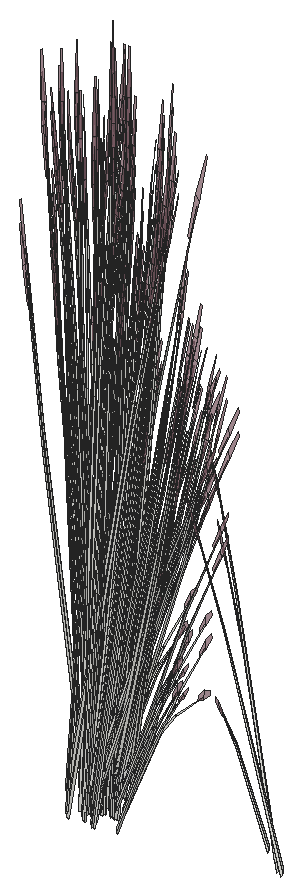
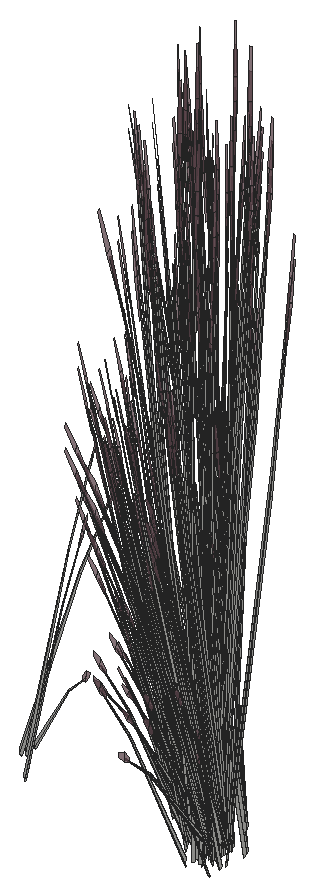
# SketchUp Ruby script. Lengths in inches.
U = 1.inch
M = Sketchup.active_model
def pt(a) = Geom::Point3d.new(a.map { |v| v * U })
def face(e, loops, mat)
  f = e.add_face(loops[0].map { |a| pt(a) })
  loops[1..].each { |l| e.add_face(l.map { |a| pt(a) }).erase! }
  f.material = f.back_material = mat if mat
  f
end
# faces: each face lists its corners as indices into pts; further lists are holes
def faces(e, pts, list, mat = nil) = list.each { |f| face(e, (f[0].is_a?(Array) ? f : [f]).map { |l| l.map { |i| pts[i] } }, mat) }
# xy, xz, yz: faces in a plane at the given z, y or x. An outline is a flat list of corners, or four numbers for a rectangle; further outlines are holes
def ring(l) = l.size == 4 ? [[l[0], l[1]], [l[2], l[1]], [l[2], l[3]], [l[0], l[3]]] : l.each_slice(2).to_a
def flat(e, list, mat, &to3) = list.each { |f| face(e, (f[0].is_a?(Array) ? f : [f]).map { |l| ring(l).map { |u, v| to3.(u, v) } }, mat) }
def xy(e, z, list, mat = nil) = flat(e, list, mat) { |x, y| [x, y, z] }
def xz(e, y, list, mat = nil) = flat(e, list, mat) { |x, z| [x, y, z] }
def yz(e, x, list, mat = nil) = flat(e, list, mat) { |y, z| [x, y, z] }
def lines(e, pts, list) = list.each { |a, b| e.add_line(pt(pts[a]), pt(pts[b])) }
# prism: a flat outline (further loops are holes) pulled along v
def prism(e, loops, v, mat = nil)
  f = face(e, loops, mat); d = Geom::Vector3d.new(v.map { |x| x * U })
  f.pushpull(f.normal.samedirection?(d) ? d.length : -d.length)
end
def box(e, o, s, mat = nil) = prism(e, [[o, [o[0] + s[0], o[1], o[2]], [o[0] + s[0], o[1] + s[1], o[2]], [o[0], o[1] + s[1], o[2]]]], [0, 0, s[2]], mat)
def at(x, y, z, deg = 0) = Geom::Transformation.translation(pt([x, y, z])) * Geom::Transformation.rotation(ORIGIN, Z_AXIS, deg.degrees)
def axes(o, x, y, z) = Geom::Transformation.new([*x, 0, *y, 0, *z, 0, *pt(o).to_a, 1])
def part(name) = M.definitions.add(name)
# library, detail: a bought-in or finely detailed component or shape, given as its bounding box
def library(name, o, s) = part(name).tap { |d| box(d.entities, o, s) }
def detail(e, o, s) = box(e.add_group.entities, o, s)
def put(e, d, t, mat = nil) = e.add_instance(d, t).tap { |i| i.material = mat if mat }
def group(e, t, mat = nil) = e.add_group.tap { |g| g.transformation = t; g.material = mat if mat }.entities
root = M.entities
M.materials.add("LightPink_Translucent").color = [144, 107, 117]
M.materials["LightPink_Translucent"].alpha = 0.75
c1 = part("blade")
p = [[2.15,0.21,22],[0,0.17,0],[0.09,0.45,0],[2.18,0.31,22],[2.29,0.31,22],[0.38,0.45,0],
  [2.48,0.24,33],[2.49,0.24,33],[2.48,0.22,33]]
faces(c1.entities,p,[[0,1,2,3],[4,5,2,3],[6,3,4,7],[8,0,3,6]])
c2 = part("seeds")
p = [[0.3,-0.1,1.38],[-0.01,-0.03,1.59],[-0.01,-0.03,0.03],[0.14,-0.07,-0.07],[0.29,-0.03,3],[0.15,0.01,3.11]]
faces(c2.entities,p,[[0,1,2,3],[1,0,4,5]],"LightPink_Translucent")
c3 = part("blade with seeds")
put(c3.entities,c1,at(0,0,0))
put(c3.entities,c2,axes([2.4,0.25,30.99],[1.5799,-0.05474,1.17369],[-0.12525,1.92788,0.29478],[-0.07173,-0.02425,1.56792]))
put(root,c3,axes([274.08,462.69,652.73],[-0.35779,-0.36745,0.48003],[0.37996,-0.3169,0.3958],[-0.066,0.17239,0.9933]))
put(root,c3,axes([274.34,462.3125,650.03],[-0.11803,-0.46926,-0.30978],[0.46876,-0.13325,0.30978],[-0.0945,-0.05411,1.38974]))
put(root,c3,axes([274.34,462.3125,652.03],[-0.11803,-0.46926,-0.30978],[0.46876,-0.13325,0.30978],[-0.0945,-0.05411,1.38974]))
put(root,c3,axes([273.95,462.66,652.73],[-0.4129,-0.02509,0.0643],[0.01132,-0.37891,0.50621],[-0.04321,0.14514,0.77189]))
put(root,c3,axes([274.08,462.8,652.53],[-0.33997,0.28354,-0.35414],[-0.32182,-0.32376,0.4572],[-0.04897,0.1645,0.87481]))
put(root,c3,axes([274.08,462.8,654.53],[-0.33997,0.28354,-0.35414],[-0.32182,-0.32376,0.4572],[-0.04897,0.1645,0.87481]))
put(root,c3,axes([275.82,461.95,650.06],[-0.33843,0.40479,-0.62353],[-0.42041,-0.36705,-0.16365],[-0.13561,0.10098,1.37633]))
put(root,c3,axes([275.82,461.95,652.06],[-0.33843,0.40479,-0.62353],[-0.42041,-0.36705,-0.16365],[-0.13561,0.10098,1.37633]))
put(root,c3,axes([272.87,463.8125,652.71],[0.057,-0.03251,1.77383],[0.47114,0.21627,-0.16761],[-0.01107,0.18007,0.31391]))
put(root,c3,axes([276.05,461.73,650.46],[-0.49063,-0.43346,-0.25192],[0.41285,-0.48673,0.5513],[-0.13212,0.05071,1.68216]))
put(root,c3,axes([276.05,461.73,652.46],[-0.49063,-0.43346,-0.25192],[0.41285,-0.48673,0.5513],[-0.13212,0.05071,1.68216]))
put(root,c3,axes([274.31,462.5,653.34],[-0.01307,0.49815,-0.7886],[-0.55054,-0.03346,0.09517],[-0.0581,0.21104,1.11556]))
put(root,c3,axes([274.31,462.5,655.34],[-0.01307,0.49815,-0.7886],[-0.55054,-0.03346,0.09517],[-0.0581,0.21104,1.11556]))
put(root,c3,axes([274.3,463.9,650.77],[-0.013,-0.32022,1.1486],[0.32493,0.22839,0.84392],[-0.0639,0.15263,0.25299]))
put(root,c3,axes([274.3,463.9,652.77],[-0.013,-0.32022,1.1486],[0.32493,0.22839,0.84392],[-0.0639,0.15263,0.25299]))
put(root,c3,axes([275.8,461.63,650.21],[-0.54562,0.03324,-0.44739],[-0.04934,-0.55185,0.21531],[-0.09768,0.05593,1.43643]))
put(root,c3,axes([275.8,461.63,652.21],[-0.54562,0.03324,-0.44739],[-0.04934,-0.55185,0.21531],[-0.09768,0.05593,1.43643]))
put(root,c3,axes([274.76,462.56,650.48],[0.47024,0.26927,0.49651],[-0.28107,0.48284,0],[-0.1071,-0.06133,1.57504]))
put(root,c3,axes([274.76,462.56,652.48],[0.47024,0.26927,0.49651],[-0.28107,0.48284,0],[-0.1071,-0.06133,1.57504]))
put(root,c3,axes([274.12,463.2,651.36],[0.01104,-0.27801,1.54345],[0.49652,0.14685,0.21329],[-0.04302,0.2963,0.72882]))
put(root,c3,axes([274.12,463.2,653.36],[0.01104,-0.27801,1.54345],[0.49652,0.14685,0.21329],[-0.04302,0.2963,0.72882]))
put(root,c3,axes([275.44,461.72,650.62],[-0.09693,0.48062,0.1448],[-0.47357,-0.08343,-0.41347],[-0.08619,-0.04935,1.26744]))
put(root,c3,axes([275.44,461.72,652.62],[-0.09693,0.48062,0.1448],[-0.47357,-0.08343,-0.41347],[-0.08619,-0.04935,1.26744]))
put(root,c3,axes([276.38,463.06,650.02],[-0.47024,0.26927,-0.49651],[-0.28107,-0.48284,0],[-0.1071,0.06133,1.57504]))
put(root,c3,axes([276.38,463.06,652.02],[-0.47024,0.26927,-0.49651],[-0.28107,-0.48284,0],[-0.1071,0.06133,1.57504]))
put(root,c3,axes([276.41,462.91,650.19],[-0.31023,-0.54153,-0.05142],[0.52557,-0.30095,0.51607],[-0.12951,0.05156,1.6363]))
put(root,c3,axes([276.41,462.91,652.19],[-0.31023,-0.54153,-0.05142],[0.52557,-0.30095,0.51607],[-0.12951,0.05156,1.6363]))
put(root,c3,axes([274.42,462.67,653],[0.35968,0.36185,-0.5672],[-0.37996,0.3169,-0.43934],[-0.05473,0.18385,1.08528]))
put(root,c3,axes([274.42,462.67,655],[0.35968,0.36185,-0.5672],[-0.37996,0.3169,-0.43934],[-0.05473,0.18385,1.08528]))
put(root,c3,axes([276.27,462.84,650.03],[-0.46876,-0.13325,-0.30978],[0.11803,-0.46926,0.30978],[-0.0945,0.05411,1.38974]))
put(root,c3,axes([276.27,462.84,652.03],[-0.46876,-0.13325,-0.30978],[0.11803,-0.46926,0.30978],[-0.0945,0.05411,1.38974]))
put(root,c3,axes([274.26,462.4,653.05],[0.33997,-0.28354,0.35414],[0.32182,0.32376,-0.4572],[-0.04897,0.1645,0.87481]))
put(root,c3,axes([276.54,460.84,650.84],[-0.01373,-0.50706,1.41272],[0.62119,0.13144,0.59816],[-0.14692,0.27746,1.3335]))
put(root,c3,axes([276.54,460.84,652.84],[-0.01373,-0.50706,1.41272],[0.62119,0.13144,0.59816],[-0.14692,0.27746,1.3335]))
put(root,c3,axes([274.04,462.48,653.4],[0.55221,0.02668,-0.13498],[-0.01509,0.50521,-0.74919],[-0.03836,0.19458,1.13838]))
put(root,c3,axes([274.03,463.21,650.82],[0.45645,-0.09537,0.06507],[0.10494,0.38421,-0.86304],[-0.02894,0.19449,0.7736]))
put(root,c3,axes([274.03,463.21,652.82],[0.45645,-0.09537,0.06507],[0.10494,0.38421,-0.86304],[-0.02894,0.19449,0.7736]))
put(root,c3,axes([276.1875,461.48,650.67],[0.05855,0.61451,-0.29095],[-0.60981,0.03716,-0.50002],[-0.10738,0.08185,1.59708]))
put(root,c3,axes([276.1875,461.48,652.67],[0.05855,0.61451,-0.29095],[-0.60981,0.03716,-0.50002],[-0.10738,0.08185,1.59708]))
put(root,c3,axes([274.83,462.15,651.875],[-0.0123,-0.2067,1.71376],[0.53301,0.13712,0.13857],[-0.03297,0.29456,0.73262]))
put(root,c3,axes([274.83,462.15,653.875],[-0.0123,-0.2067,1.71376],[0.53301,0.13712,0.13857],[-0.03297,0.29456,0.73262]))
put(root,c3,axes([275.28,461.26,650.36],[0.63506,0.11347,0.45755],[-0.12924,0.64083,0.17955],[-0.09281,-0.06188,1.58856]))
put(root,c3,axes([275.28,461.26,652.36],[0.63506,0.11347,0.45755],[-0.12924,0.64083,0.17955],[-0.09281,-0.06188,1.58856]))
put(root,c3,axes([275.11,461.14,650.72],[-0.24378,0.48527,0.44739],[-0.50654,-0.23354,-0.21531],[0,-0.11186,1.43643]))
put(root,c3,axes([275.11,461.14,652.72],[-0.24378,0.48527,0.44739],[-0.50654,-0.23354,-0.21531],[0,-0.11186,1.43643]))
put(root,c3,axes([274.9375,462.28,650.47],[0.53992,-0.14294,0.17642],[0.13332,0.53195,0.35086],[-0.04815,-0.07751,1.60407]))
put(root,c3,axes([274.9375,462.28,652.47],[0.53992,-0.14294,0.17642],[0.13332,0.53195,0.35086],[-0.04815,-0.07751,1.60407]))
put(root,c3,axes([275.63,462.37,650.2],[-0.50654,-0.24178,0],[0.24378,-0.50239,0],[0,0,1.62707]))
put(root,c3,axes([275.63,462.37,652.2],[-0.50654,-0.24178,0],[0.24378,-0.50239,0],[0,0,1.62707]))
put(root,c3,axes([276.8,462.97,650.375],[0.31414,0.53965,0],[-0.52557,0.30095,-0.51607],[-0.1197,0.06854,1.63711]))
put(root,c3,axes([276.8,462.97,652.375],[0.31414,0.53965,0],[-0.52557,0.30095,-0.51607],[-0.1197,0.06854,1.63711]))
put(root,c3,axes([275.21,463.21,653.0625],[-0.4951,-0.14079,0.53283],[0.1693,-0.46287,0.43934],[0.02975,0.18203,1.10256]))
put(root,c3,axes([275.07,463.24,652.73],[-0.37023,0.18303,0.0643],[-0.18122,-0.33376,0.50621],[0.03575,0.14712,0.77189]))
put(root,c3,axes([276.54,462.3125,650.47],[0.14515,-0.53522,0.17642],[0.53115,0.15146,0.35086],[-0.09175,0.00261,1.60407]))
put(root,c3,axes([276.54,462.3125,652.47],[0.14515,-0.53522,0.17642],[0.53115,0.15146,0.35086],[-0.09175,0.00261,1.60407]))
put(root,c3,axes([276.3,461.6,650.62],[0.37121,0.32357,0.1448],[-0.30963,0.36505,-0.41347],[-0.08619,0.04935,1.26744]))
put(root,c3,axes([276.3,461.6,652.62],[0.37121,0.32357,0.1448],[-0.30963,0.36505,-0.41347],[-0.08619,0.04935,1.26744]))
put(root,c3,axes([276.17,461.2,650.3],[-0.46736,-0.46353,-0.06131],[0.46764,-0.46381,0],[-0.01632,-0.01619,1.75571]))
put(root,c3,axes([276.17,461.2,652.3],[-0.46736,-0.46353,-0.06131],[0.46764,-0.46381,0],[-0.01632,-0.01619,1.75571]))
put(root,c3,axes([276.29,461.37,650.72],[0.54562,-0.03324,0.44739],[0.04934,0.55185,-0.21531],[-0.09768,0.05593,1.43643]))
put(root,c3,axes([276.29,461.37,652.72],[0.54562,-0.03324,0.44739],[0.04934,0.55185,-0.21531],[-0.09768,0.05593,1.43643]))
put(root,c3,axes([276.42,462.63,650.33],[0.62903,0.17504,0.30756],[-0.15737,0.62568,-0.36492],[-0.10411,0.07831,1.64885]))
put(root,c3,axes([276.42,462.63,652.33],[0.62903,0.17504,0.30756],[-0.15737,0.62568,-0.36492],[-0.10411,0.07831,1.64885]))
put(root,c3,axes([276.69,462.6,650.48],[0.47024,-0.26927,0.49651],[0.28107,0.48284,0],[-0.1071,0.06133,1.57504]))
put(root,c3,axes([276.69,462.6,652.48],[0.47024,-0.26927,0.49651],[0.28107,0.48284,0],[-0.1071,0.06133,1.57504]))
put(root,c3,axes([275.75,462.16,650.2],[-0.16394,-0.4643,0],[0.46814,-0.1626,0],[0,0,1.54371]))
put(root,c3,axes([275.75,462.16,652.2],[-0.16394,-0.4643,0],[0.46814,-0.1626,0],[0,0,1.54371]))
put(root,c3,axes([275.15,463.14,649.49],[0.08132,-0.0293,1.76342],[0.48914,0.1613,-0.26939],[0.0143,0.18179,0.30037]))
put(root,c3,axes([275.15,463.14,651.49],[0.08132,-0.0293,1.76342],[0.48914,0.1613,-0.26939],[0.0143,0.18179,0.30037]))
put(root,c3,axes([275.26,463.3,652.53],[-0.15148,0.41415,-0.35414],[-0.44193,-0.12079,0.4572],[0.04052,0.16674,0.87481]))
put(root,c3,axes([275.26,463.3,654.53],[-0.15148,0.41415,-0.35414],[-0.44193,-0.12079,0.4572],[0.04052,0.16674,0.87481]))
put(root,c3,axes([276.41,461.24,650.21],[-0.24378,0.48527,-0.44739],[-0.50654,-0.23354,0.21531],[0,0.11186,1.43643]))
put(root,c3,axes([276.41,461.24,652.21],[-0.24378,0.48527,-0.44739],[-0.50654,-0.23354,0.21531],[0,0.11186,1.43643]))
put(root,c3,axes([274.95,464.04,652.72],[0.06369,0.08672,1.74944],[0.51399,0.03407,-0.27667],[0.05169,0.19126,0.14031]))
put(root,c3,axes([277.375,460.95,650.47],[-0.39477,-0.39228,0.17642],[0.39783,-0.38049,0.35086],[-0.0436,0.08011,1.60407]))
put(root,c3,axes([277.375,460.95,652.47],[-0.39477,-0.39228,0.17642],[0.39783,-0.38049,0.35086],[-0.0436,0.08011,1.60407]))
put(root,c3,axes([276.01,460.72,650.21],[0,-0.62313,0],[0.62828,0,0],[0,0,1.79456]))
put(root,c3,axes([276.01,460.72,652.21],[0,-0.62313,0],[0.62828,0,0],[0,0,1.79456]))
put(root,c3,axes([276.33,460.97,650.29],[0,0.62282,-0.05637],[-0.62828,0,0],[0,0.01957,1.79368]))
put(root,c3,axes([276.33,460.97,652.29],[0,0.62282,-0.05637],[-0.62828,0,0],[0,0.01957,1.79368]))
put(root,c3,axes([275.21,462.87,653.05],[0.15148,-0.41415,0.35414],[0.44193,0.12079,-0.4572],[0.04052,0.16674,0.87481]))
put(root,c3,axes([274.99,459.52,650.47],[-0.14515,0.53522,0.17642],[-0.53115,-0.15146,0.35086],[0.09175,-0.00261,1.60407]))
put(root,c3,axes([274.99,459.52,652.47],[-0.14515,0.53522,0.17642],[-0.53115,-0.15146,0.35086],[0.09175,-0.00261,1.60407]))
put(root,c3,axes([276.03,462.18,650.29],[0.21845,0.61869,-0.06012],[-0.62418,0.21679,0],[0.00763,0.02161,1.72173]))
put(root,c3,axes([276.03,462.18,652.29],[0.21845,0.61869,-0.06012],[-0.62418,0.21679,0],[0.00763,0.02161,1.72173]))
put(root,c3,axes([275.31,462.93,652.98],[0.23981,0.43789,-0.71045],[-0.49365,0.24404,0.08574],[0.05608,0.21158,1.00501]))
put(root,c3,axes([275.31,462.93,654.98],[0.23981,0.43789,-0.71045],[-0.49365,0.24404,0.08574],[0.05608,0.21158,1.00501]))
put(root,c3,axes([277.83,461.36,650.2],[-0.62797,-0.00431,-0.04976],[0,-0.6019,0.49943],[-0.01973,0.13702,1.58352]))
put(root,c3,axes([277.83,461.36,652.2],[-0.62797,-0.00431,-0.04976],[0,-0.6019,0.49943],[-0.01973,0.13702,1.58352]))
put(root,c3,axes([276.6,459.55,650.47],[-0.53992,0.14294,0.17642],[-0.13332,-0.53195,0.35086],[0.04815,0.07751,1.60407]))
put(root,c3,axes([276.6,459.55,652.47],[-0.53992,0.14294,0.17642],[-0.13332,-0.53195,0.35086],[0.04815,0.07751,1.60407]))
put(root,c3,axes([275.81,464.34,653.65],[0.34721,-0.30895,-0.06488],[0.31814,0.33837,-0.29416],[0.0224,0.09588,0.97024]))
put(root,c3,axes([275.71,460.33,650.36],[-0.4166,0.48873,0.45755],[-0.49494,-0.43142,0.17955],[0.10044,-0.04877,1.58856]))
put(root,c3,axes([275.71,460.33,652.36],[-0.4166,0.48873,0.45755],[-0.49494,-0.43142,0.17955],[0.10044,-0.04877,1.58856]))
put(root,c3,axes([276.42,461.1,650.21],[0.35073,0.34786,0],[-0.35073,0.34786,0],[0,0,1.69266]))
put(root,c3,axes([276.42,461.1,652.21],[0.35073,0.34786,0],[-0.35073,0.34786,0],[0,0,1.69266]))
put(root,c3,axes([276.42,460.69,650.72],[0.24378,-0.48527,0.44739],[0.50654,0.23354,-0.21531],[0,0.11186,1.43643]))
put(root,c3,axes([276.42,460.69,652.72],[0.24378,-0.48527,0.44739],[0.50654,0.23354,-0.21531],[0,0.11186,1.43643]))
put(root,c3,axes([276.21,462.38,650.2],[0.50654,0.24178,0],[-0.24378,0.50239,0],[0,0,1.74954]))
put(root,c3,axes([276.21,462.38,652.2],[0.50654,0.24178,0],[-0.24378,0.50239,0],[0,0,1.74954]))
put(root,c3,axes([275.49,463.02,652.68],[0.49392,0.135,-0.51099],[-0.1693,0.46287,-0.3958],[0.04529,0.18636,0.97773]))
put(root,c3,axes([275.49,463.02,654.68],[0.49392,0.135,-0.51099],[-0.1693,0.46287,-0.3958],[0.04529,0.18636,0.97773]))
put(root,c3,axes([275.0625,463.04,653.03],[0.49168,-0.25073,-0.1216],[0.24162,0.44501,-0.67495],[0.06487,0.18753,1.02557]))
put(root,c3,axes([276.25,460.58,650.38],[-0.63506,-0.11347,0.49198],[0.12924,-0.64083,0.19306],[0.09281,0.06188,1.70813]))
put(root,c3,axes([276.25,460.58,652.38],[-0.63506,-0.11347,0.49198],[0.12924,-0.64083,0.19306],[0.09281,0.06188,1.70813]))
put(root,c3,axes([277.7,461.45,650.03],[-0.35073,0.33601,-0.30978],[-0.35073,-0.33601,0.30978],[0,0.10823,1.38974]))
put(root,c3,axes([277.7,461.45,652.03],[-0.35073,0.33601,-0.30978],[-0.35073,-0.33601,0.30978],[0,0.10823,1.38974]))
put(root,c3,axes([276.7,461.39,650.09],[0.18424,0.49308,-0.69212],[-0.53071,0.17758,-0.18165],[0.02036,0.16697,1.52773]))
put(root,c3,axes([276.7,461.39,652.09],[0.18424,0.49308,-0.69212],[-0.53071,0.17758,-0.18165],[0.02036,0.16697,1.52773]))
put(root,c3,axes([276.4375,460.86,650.21],[0.56215,0,0],[0,0.55754,0],[0,0,1.78407]))
put(root,c3,axes([276.4375,460.86,652.21],[0.56215,0,0],[0,0.55754,0],[0,0,1.78407]))
put(root,c3,axes([275.9,460.25,650.72],[-0.30184,-0.45202,0.44739],[0.45719,-0.31831,-0.21531],[0.09768,0.05593,1.43643]))
put(root,c3,axes([275.9,460.25,652.72],[-0.30184,-0.45202,0.44739],[0.45719,-0.31831,-0.21531],[0.09768,0.05593,1.43643]))
put(root,c3,axes([276.63,460.8,650.62],[0.46814,-0.15705,0.1448],[0.16394,0.44848,-0.41347],[0,0.0987,1.26744]))
put(root,c3,axes([276.63,460.8,652.62],[0.46814,-0.15705,0.1448],[0.16394,0.44848,-0.41347],[0,0.0987,1.26744]))
put(root,c3,axes([276.47,460.84,650.67],[0.56585,0.25696,-0.29095],[-0.27246,0.54236,-0.50002],[0.01778,0.13316,1.59708]))
put(root,c3,axes([276.47,460.84,652.67],[0.56585,0.25696,-0.29095],[-0.27246,0.54236,-0.50002],[0.01778,0.13316,1.59708]))
put(root,c3,axes([277.7,460.96,650.48],[0,-0.53854,0.49651],[0.56215,0,0],[0,0.12266,1.57504]))
put(root,c3,axes([277.7,460.96,652.48],[0,-0.53854,0.49651],[0.56215,0,0],[0,0.12266,1.57504]))
put(root,c3,axes([277.94,461.46,650.02],[0,0.53854,-0.49651],[-0.56215,0,0],[0,0.12266,1.57504]))
put(root,c3,axes([277.94,461.46,652.02],[0,0.53854,-0.49651],[-0.56215,0,0],[0,0.12266,1.57504]))
put(root,c3,axes([276.4375,463.09,652.73],[-0.49974,0.12359,0.48003],[-0.08673,-0.48481,0.3958],[0.11753,0.14288,0.9933]))
put(root,c3,axes([276.34,463.19,652.73],[-0.22836,0.34211,0.0643],[-0.3252,-0.19918,0.50621],[0.10513,0.10968,0.77189]))
put(root,c3,axes([275.77,462.0625,651.875],[-0.11485,-0.17291,1.71376],[0.53072,-0.14557,0.13857],[0.11995,0.27145,0.73262]))
put(root,c3,axes([275.77,462.0625,653.875],[-0.11485,-0.17291,1.71376],[0.53072,-0.14557,0.13857],[0.11995,0.27145,0.73262]))
put(root,c3,axes([276.1,460.12,650.62],[0.09693,-0.48062,0.1448],[0.47357,0.08343,-0.41347],[0.08619,0.04935,1.26744]))
put(root,c3,axes([276.1,460.12,652.62],[0.09693,-0.48062,0.1448],[0.47357,0.08343,-0.41347],[0.08619,0.04935,1.26744]))
put(root,c3,axes([276.77,459.28,650.48],[-0.47024,-0.26927,0.49651],[0.28107,-0.48284,0],[0.1071,0.06133,1.57504]))
put(root,c3,axes([276.77,459.28,652.48],[-0.47024,-0.26927,0.49651],[0.28107,-0.48284,0],[0.1071,0.06133,1.57504]))
put(root,c3,axes([276.36,462.09,650.18],[0.5275,-0.18273,-0.19198],[0.18536,0.52636,0.00008],[0.05823,-0.0202,1.73897]))
put(root,c3,axes([276.36,462.09,652.18],[0.5275,-0.18273,-0.19198],[0.18536,0.52636,0.00008],[0.05823,-0.0202,1.73897]))
put(root,c3,axes([276.27,462.8,653.05],[-0.0776,-0.43378,0.35414],[0.44361,-0.11454,-0.4572],[0.11915,0.12431,0.87481]))
put(root,c3,axes([276.37,460.53,650.21],[0.30184,0.45202,-0.44739],[-0.45719,0.31831,0.21531],[0.09768,0.05593,1.43643]))
put(root,c3,axes([276.37,460.53,652.21],[0.30184,0.45202,-0.44739],[-0.45719,0.31831,0.21531],[0.09768,0.05593,1.43643]))
put(root,c3,axes([276.57,460.3,652.47],[-0.43417,-0.27982,1.38283],[0.45844,-0.43566,0.59665],[0.14008,0.26255,1.33663]))
put(root,c3,axes([275.84,463.4,652.71],[0.00149,-0.0652,1.77383],[0.43058,-0.28766,-0.16761],[0.14956,0.10267,0.31391]))
put(root,c3,axes([277.23,462.58,650.77],[-0.2829,-0.15485,1.1486],[0.36529,-0.15734,0.84392],[0.09853,0.13328,0.25299]))
put(root,c3,axes([277.23,462.58,652.77],[-0.2829,-0.15485,1.1486],[0.36529,-0.15734,0.84392],[0.09853,0.13328,0.25299]))
put(root,c3,axes([276.22,462.41,650.59],[0.00887,-0.17852,1.43002],[0.42372,-0.19941,-0.30754],[0.1308,0.21367,0.61141]))
put(root,c3,axes([276.22,462.41,652.59],[0.00887,-0.17852,1.43002],[0.42372,-0.19941,-0.30754],[0.1308,0.21367,0.61141]))
put(root,c3,axes([277.2,459.53,650.03],[0.11803,0.46926,-0.30978],[-0.46876,0.13325,0.30978],[0.0945,0.05411,1.38974]))
put(root,c3,axes([277.2,459.53,652.03],[0.11803,0.46926,-0.30978],[-0.46876,0.13325,0.30978],[0.0945,0.05411,1.38974]))
put(root,c3,axes([278.08,461.05,650.375],[0.62828,0,0],[0,0.6019,-0.51607],[0,0.13709,1.63711]))
put(root,c3,axes([278.08,461.05,652.375],[0.62828,0,0],[0,0.6019,-0.51607],[0,0.13709,1.63711]))
put(root,c3,axes([276.05,460.27,650.67],[0.5073,-0.35754,-0.29095],[0.33735,0.5052,-0.50002],[0.12516,0.05131,1.59708]))
put(root,c3,axes([276.05,460.27,652.67],[0.5073,-0.35754,-0.29095],[0.33735,0.5052,-0.50002],[0.12516,0.05131,1.59708]))
put(root,c3,axes([277.27,463.28,650.67],[-0.3222,-0.01689,1.0506],[0.21278,-0.35872,0.58006],[0.12729,0.12745,0.8241]))
put(root,c3,axes([277.27,463.28,652.67],[-0.3222,-0.01689,1.0506],[0.21278,-0.35872,0.58006],[0.12729,0.12745,0.8241]))
put(root,c3,axes([276.23,463.02,653.03],[0.2994,-0.46097,-0.1216],[0.43359,0.26557,-0.67495],[0.15072,0.13024,1.02557]))
put(root,c3,axes([274.77,459.96,649.59],[-0.49456,0.21561,1.28929],[-0.15741,-0.61865,0.50096],[0.30369,0.01029,1.46642]))
put(root,c3,axes([274.77,459.96,651.59],[-0.49456,0.21561,1.28929],[-0.15741,-0.61865,0.50096],[0.30369,0.01029,1.46642]))
put(root,c3,axes([276.59,462.79,652.68],[0.4958,-0.12802,-0.51099],[0.08673,0.48481,-0.3958],[0.13317,0.13893,0.97773]))
put(root,c3,axes([276.59,462.79,654.68],[0.4958,-0.12802,-0.51099],[0.08673,0.48481,-0.3958],[0.13317,0.13893,0.97773]))
put(root,c3,axes([277.16,462.21,653.05],[-0.28589,-0.33718,0.35414],[0.32644,-0.31919,-0.4572],[0.16586,0.04856,0.87481]))
put(root,c3,axes([277.33,459.32,650.02],[0.47024,0.26927,-0.49651],[-0.28107,0.48284,0],[0.1071,0.06133,1.57504]))
put(root,c3,axes([277.33,459.32,652.02],[0.47024,0.26927,-0.49651],[-0.28107,0.48284,0],[0.1071,0.06133,1.57504]))
put(root,c3,axes([277.42,462.52,652.73],[-0.0253,0.40952,0.0643],[-0.38204,-0.01123,0.50621],[0.14634,0.04285,0.77189]))
put(root,c3,axes([277.31,463.16,649.49],[0.03661,-0.07775,1.76342],[0.46087,-0.22898,-0.26939],[0.13972,0.11851,0.30037]))
put(root,c3,axes([277.31,463.16,651.49],[0.03661,-0.07775,1.76342],[0.46087,-0.22898,-0.26939],[0.13972,0.11851,0.30037]))
put(root,c3,axes([277.45,462.39,652.73],[-0.37048,0.35486,0.48003],[-0.31952,-0.37685,0.3958],[0.17382,0.06546,0.9933]))
put(root,c3,axes([278.41,462.4375,651.93],[-0.09617,-0.45271,-0.03492],[0.45453,-0.10408,-0.15832],[0.09492,0.0287,0.52218]))
put(root,c3,axes([278.41,462.4375,653.93],[-0.09617,-0.45271,-0.03492],[0.45453,-0.10408,-0.15832],[0.09492,0.0287,0.52218]))
put(root,c3,axes([277.625,461.27,653.05],[-0.41757,-0.15024,0.35414],[0.12179,-0.4383,-0.4572],[0.16812,-0.04019,0.87481]))
put(root,c3,axes([276.64,460.36,650.06],[0.52267,0.08829,-0.62353],[-0.11029,0.54463,-0.16365],[0.15598,0.06599,1.37633]))
put(root,c3,axes([276.64,460.36,652.06],[0.52267,0.08829,-0.62353],[-0.11029,0.54463,-0.16365],[0.15598,0.06599,1.37633]))
put(root,c3,axes([276.53,461.52,651.875],[-0.18664,-0.09279,1.71376],[0.38624,-0.38925,0.13857],[0.24072,0.1756,0.73262]))
put(root,c3,axes([276.53,461.52,653.875],[-0.18664,-0.09279,1.71376],[0.38624,-0.38925,0.13857],[0.24072,0.1756,0.73262]))
put(root,c3,axes([278.01,461.4,652.73],[0.18454,0.3672,0.0643],[-0.33652,0.17973,0.50621],[0.14834,-0.03546,0.77189]))
put(root,c3,axes([277.5625,462.39,652.53],[0.28589,0.33718,-0.35414],[-0.32644,0.31919,0.4572],[0.16586,0.04856,0.87481]))
put(root,c3,axes([277.5625,462.39,654.53],[0.28589,0.33718,-0.35414],[-0.32644,0.31919,0.4572],[0.16586,0.04856,0.87481]))
put(root,c3,axes([277.23,462.43,653.03],[0.0269,-0.54769,-0.1216],[0.50939,0.01497,-0.67495],[0.19618,0.03804,1.02557]))
put(root,c3,axes([277.97,461.27,652.73],[-0.14195,0.49104,0.48003],[-0.46669,-0.16791,0.3958],[0.18353,-0.02951,0.9933]))
put(root,c3,axes([277.68,462.1,652.72],[0.10779,-0.00911,1.74944],[0.29564,-0.41839,-0.27667],[0.19172,0.05523,0.14031]))
put(root,c3,axes([278.95,461.31,650.77],[-0.31044,0.08891,1.1486],[0.14613,-0.36744,0.84392],[0.16469,0.02514,0.25299]))
put(root,c3,axes([278.95,461.31,652.77],[-0.31044,0.08891,1.1486],[0.14613,-0.36744,0.84392],[0.16469,0.02514,0.25299]))
put(root,c3,axes([278.07,461.22,652.53],[0.41757,0.15024,-0.35414],[-0.12179,0.4383,0.4572],[0.16812,-0.04019,0.87481]))
put(root,c3,axes([278.07,461.22,654.53],[0.41757,0.15024,-0.35414],[-0.12179,0.4383,0.4572],[0.16812,-0.04019,0.87481]))
put(root,c3,axes([277.26,462.16,652.98],[0.50227,0.01297,-0.71045],[-0.03373,0.54602,0.08574],[0.21278,0.05762,1.00501]))
put(root,c3,axes([277.26,462.16,654.98],[0.50227,0.01297,-0.71045],[-0.03373,0.54602,0.08574],[0.21278,0.05762,1.00501]))
put(root,c3,axes([278.63,460.8,649.49],[-0.02626,-0.08176,1.76342],[0.18213,-0.47826,-0.26939],[0.18372,-0.00688,0.30037]))
put(root,c3,axes([278.63,460.8,651.49],[-0.02626,-0.08176,1.76342],[0.18213,-0.47826,-0.26939],[0.18372,-0.00688,0.30037]))
put(root,c3,axes([278.81,462.86,652.71],[-0.04543,-0.04715,1.77383],[0.09938,-0.50538,-0.16761],[0.17896,-0.03229,0.31391]))
put(root,c3,axes([276.93,460.67,651.875],[-0.20841,0.0122,1.71376],[0.13825,-0.52864,0.13857],[0.297,0.0327,0.73262]))
put(root,c3,axes([276.93,460.67,653.875],[-0.20841,0.0122,1.71376],[0.13825,-0.52864,0.13857],[0.297,0.0327,0.73262]))
put(root,c3,axes([277.69,461.17,652.98],[0.44151,-0.23785,-0.71045],[0.24605,0.4896,0.08574],[0.21333,-0.05562,1.00501]))
put(root,c3,axes([277.69,461.17,654.98],[0.44151,-0.23785,-0.71045],[0.24605,0.4896,0.08574],[0.21333,-0.05562,1.00501]))
put(root,c3,axes([278.37,461.9,650.59],[-0.12101,-0.13245,1.43002],[0.15744,-0.43816,-0.30754],[0.24483,0.05936,0.61141]))
put(root,c3,axes([278.37,461.9,652.59],[-0.12101,-0.13245,1.43002],[0.15744,-0.43816,-0.30754],[0.24483,0.05936,0.61141]))
put(root,c3,axes([293.32,461,651.875],[0.17434,-0.11391,1.71376],[0.14677,0.52637,0.13857],[-0.27369,0.11897,0.73262]))
put(root,c3,axes([292.78,461.89,650.59],[0.17462,0.04421,1.43002],[0.11254,0.45156,-0.30754],[-0.23719,0.08453,0.61141]))
put(root,c3,axes([294.33,460.45,651.34],[0.14282,-0.0779,1.77064],[0.04925,0.54394,0.13857],[-0.30935,0.07218,0.63284]))
put(root,c3,axes([292.79,460.8125,652.72],[-0.08205,0.06992,1.74944],[0.00698,0.51086,-0.27667],[-0.18807,0.06644,0.14031]))
